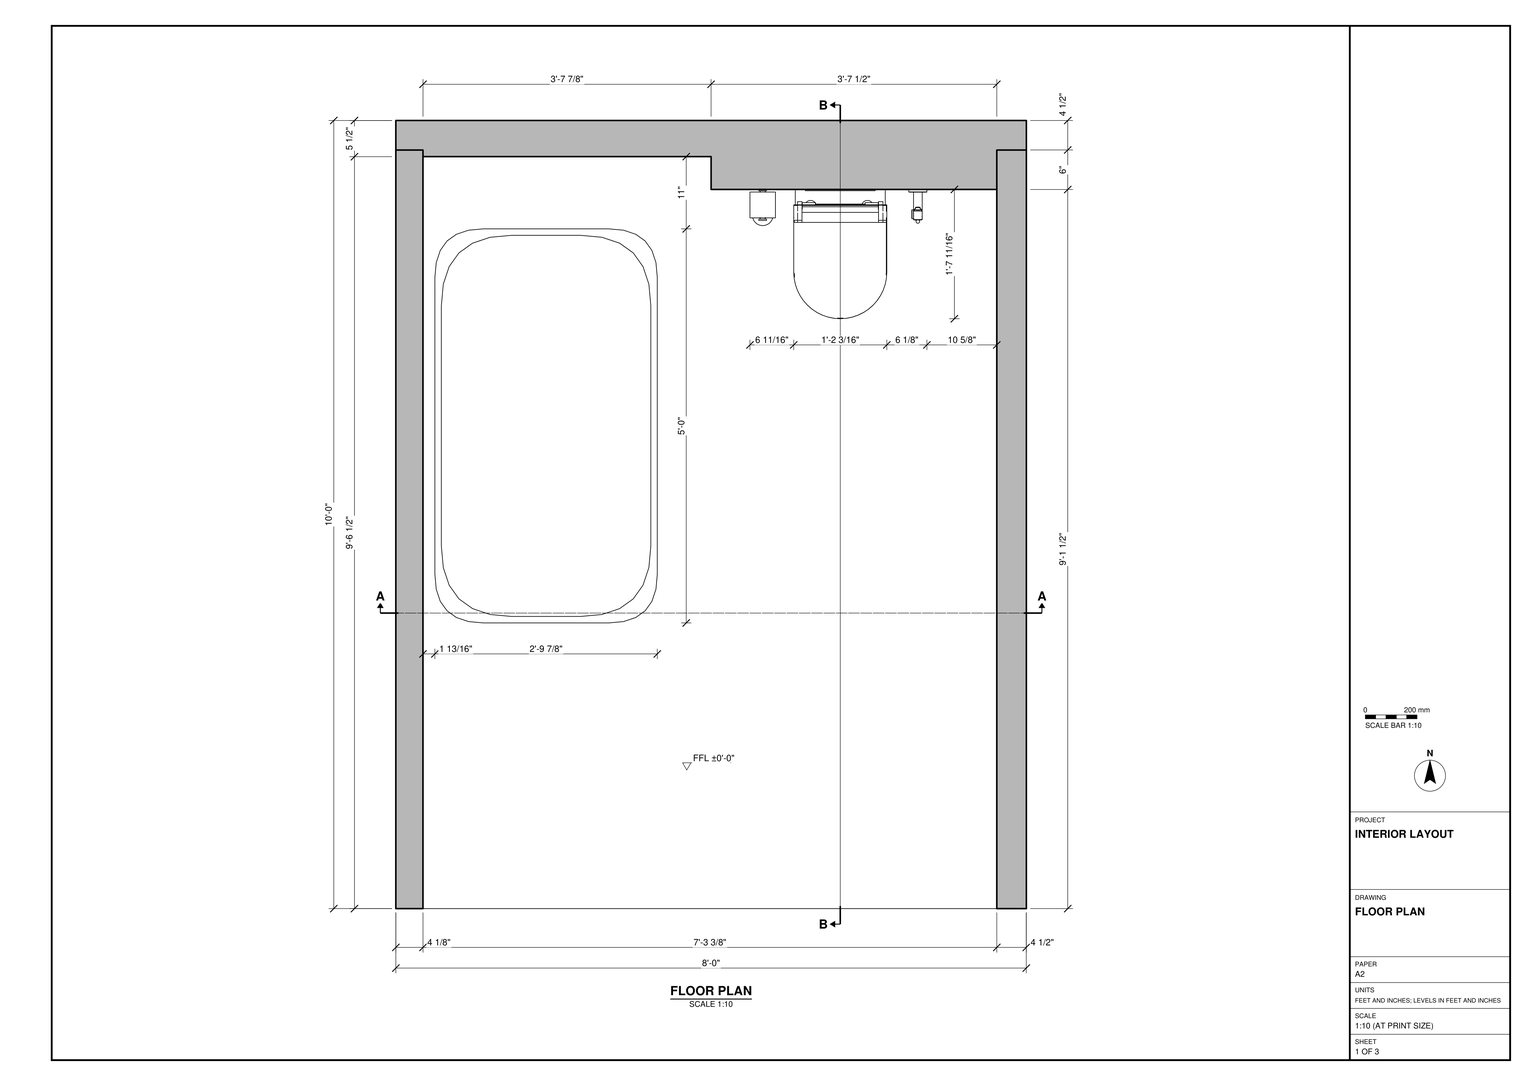
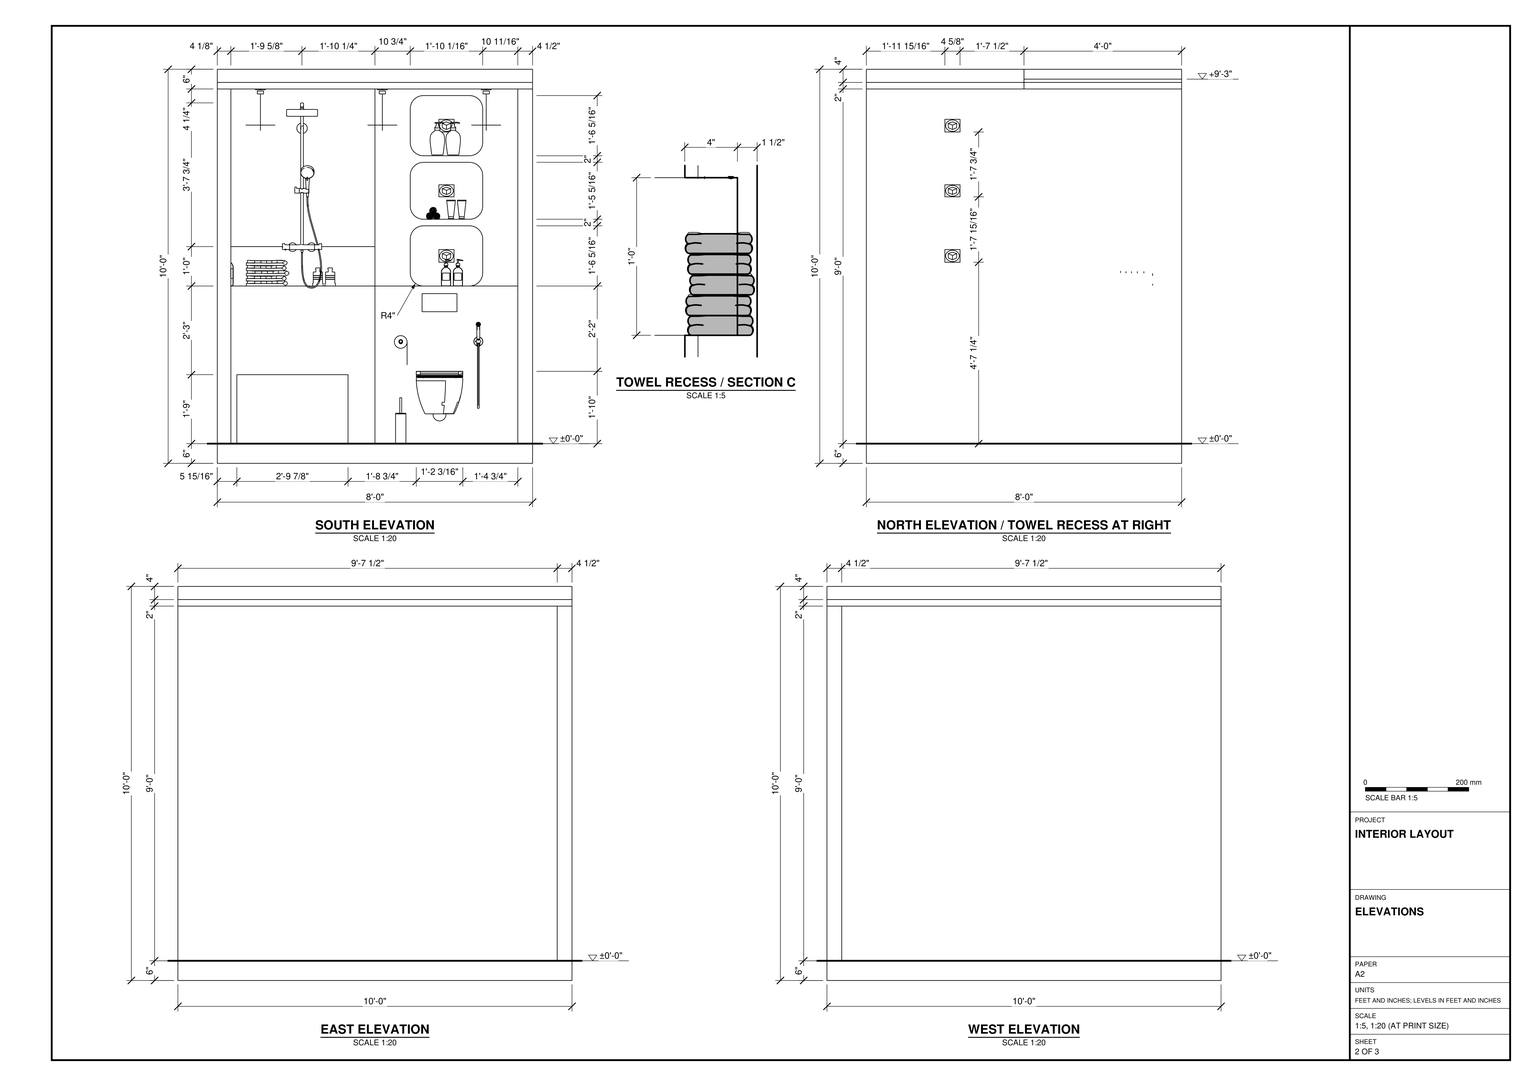
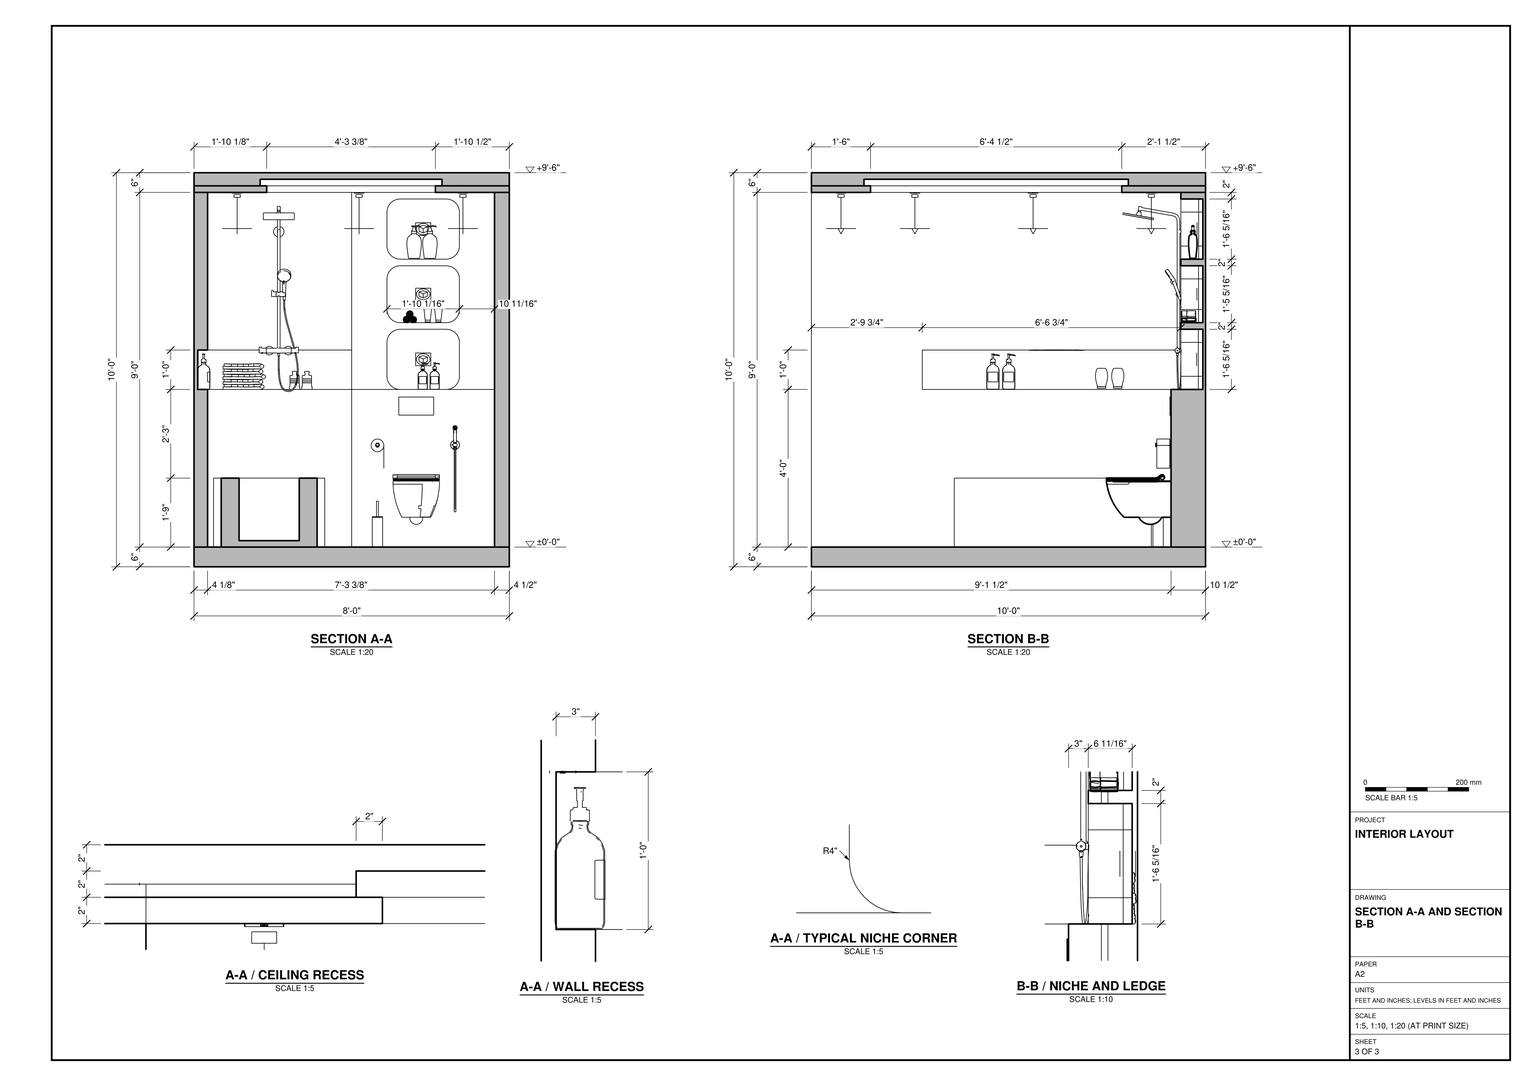
Build the bathroom in SketchUp from task_files/diagram_01.pdf. Work in feet and inches. The room shell is 8'-0" wide, 10'-0" deep and 10'-0" high overall, with the finished floor at ±0'-0". Use the plan for wall thicknesses and fixture positions, and the elevations and sections for heights and recess profiles.

Model the floor slab, the two side walls and the stepped back wall, leaving the front open as drawn. Run the bathtub lengthwise along the left wall, with a rounded rim and a hollow basin. Fit the shower head, hand shower, hose and controls at the back of the tub. Mount the toilet on the projecting part of the back wall to the right, with its flush plate above. Form the three stacked, round-cornered niches above the toilet and the horizontal storage recesses around the bathing area. Place towels and toiletries on the ledges shown. Model the stepped ceiling recess and position the ceiling lights around it as shown in section.

Keep the shell elements, fixtures and individual furniture or joinery pieces in separate groups or components, and use components for repeated parts. Decor and loose items may be any suitable library components. Save one SketchUp model as output_files/bathroom_with_a_bathtub_and_recessed_wall_storage.skp.

# SketchUp Ruby script. Lengths in inches.
U = 1.inch
M = Sketchup.active_model
def pt(a) = Geom::Point3d.new(a.map { |v| v * U })
def face(e, loops, mat)
  f = e.add_face(loops[0].map { |a| pt(a) })
  loops[1..].each { |l| e.add_face(l.map { |a| pt(a) }).erase! }
  f.material = f.back_material = mat if mat
  f
end
# faces: each face lists its corners as indices into pts; further lists are holes
def faces(e, pts, list, mat = nil) = list.each { |f| face(e, (f[0].is_a?(Array) ? f : [f]).map { |l| l.map { |i| pts[i] } }, mat) }
# xy, xz, yz: faces in a plane at the given z, y or x. An outline is a flat list of corners, or four numbers for a rectangle; further outlines are holes
def ring(l) = l.size == 4 ? [[l[0], l[1]], [l[2], l[1]], [l[2], l[3]], [l[0], l[3]]] : l.each_slice(2).to_a
def flat(e, list, mat, &to3) = list.each { |f| face(e, (f[0].is_a?(Array) ? f : [f]).map { |l| ring(l).map { |u, v| to3.(u, v) } }, mat) }
def xy(e, z, list, mat = nil) = flat(e, list, mat) { |x, y| [x, y, z] }
def xz(e, y, list, mat = nil) = flat(e, list, mat) { |x, z| [x, y, z] }
def yz(e, x, list, mat = nil) = flat(e, list, mat) { |y, z| [x, y, z] }
def lines(e, pts, list) = list.each { |a, b| e.add_line(pt(pts[a]), pt(pts[b])) }
# prism: a flat outline (further loops are holes) pulled along v
def prism(e, loops, v, mat = nil)
  f = face(e, loops, mat); d = Geom::Vector3d.new(v.map { |x| x * U })
  f.pushpull(f.normal.samedirection?(d) ? d.length : -d.length)
end
def box(e, o, s, mat = nil) = prism(e, [[o, [o[0] + s[0], o[1], o[2]], [o[0] + s[0], o[1] + s[1], o[2]], [o[0], o[1] + s[1], o[2]]]], [0, 0, s[2]], mat)
def at(x, y, z, deg = 0) = Geom::Transformation.translation(pt([x, y, z])) * Geom::Transformation.rotation(ORIGIN, Z_AXIS, deg.degrees)
def axes(o, x, y, z) = Geom::Transformation.new([*x, 0, *y, 0, *z, 0, *pt(o).to_a, 1])
def part(name) = M.definitions.add(name)
# library, detail: a bought-in or finely detailed component or shape, given as its bounding box
def library(name, o, s) = part(name).tap { |d| box(d.entities, o, s) }
def detail(e, o, s) = box(e.add_group.entities, o, s)
def put(e, d, t, mat = nil) = e.add_instance(d, t).tap { |i| i.material = mat if mat }
def group(e, t, mat = nil) = e.add_group.tap { |g| g.transformation = t; g.material = mat if mat }.entities
root = M.entities
M.materials.add("[Color M00]").color = [255, 255, 255]
c1 = library("Wall-mounted toilet",[0.42,0,-3.5625],[26.94,19.69,45.6875])
c2 = library("Component23",[-347.61,-342.26,23.58],[692.99,696.09,1706.99])
c3 = library("Component7",[-35.53,-35.9,8.59],[73.46,71.43,202.64])
c4 = library("Component24",[-60.51,-34.16,-327.68],[121.07,71.1,439.78])
c5 = library("Component25",[-33.87,-21.9,6.67],[67.74,43.8,171.96])
c6 = library("Component26",[-425.92,-315.64,5.92],[882.4,607.05,1538.44])
c7 = library("Rolled towels",[-0.87,0,-0.63],[7.91,9.92,7.86])
c8 = part("Group237\#1")
p = [[0,0,0],[0,0,-30.17],[-6.71,0,-30.17],[43.68,-54,0],[-43.68,-54,0],[43.68,54,0],
  [43.68,0,0],[-43.68,54,0],[6.71,0,-30.17],[-43.68,0,0],[0,0,-48.84]]
lines(c8.entities,p,[[0,1],[1,2],[3,4],[5,6],[7,5],[1,8],[9,0],[0,6],[8,10],[4,9],[6,3],[2,10],
  [9,7]])
c9 = part("Rectangle Light")
put(c9.entities,c8,at(0,0,0))
c10 = part("Group239\#1")
p = [[0,0,0],[0,0,-8.86],[-4.25,0,-8.86],[27.68,-1,0],[-27.68,-1,0],[27.68,1,0],
  [27.68,0,0],[-27.68,1,0],[4.25,0,-8.86],[-27.68,0,0],[0,0,-14.34]]
lines(c10.entities,p,[[0,1],[1,2],[3,4],[5,6],[7,5],[1,8],[9,0],[0,6],[8,10],[4,9],[6,3],[2,10],
  [9,7]])
c11 = part("Rectangle Light\#1")
put(c11.entities,c10,at(0,0,0))
c12 = part("Group241\#1")
p = [[0,0,0],[0,0,-12.11],[-0.15,0,-12.11],[1,-38.19,0],[-1,-38.19,0],[1,38.19,0],
  [1,0,0],[-1,38.19,0],[0.15,0,-12.11],[-1,0,0],[0,0,-19.6]]
lines(c12.entities,p,[[0,1],[1,2],[3,4],[5,6],[7,5],[1,8],[9,0],[0,6],[8,10],[4,9],[6,3],[2,10],
  [9,7]])
c13 = part("Rectangle Light\#2")
put(c13.entities,c12,at(0,0,0))
c14 = library("Mesh Light",[-0.5,-0.5,-0.1],[1,1,0.2])
c15 = library("Mesh Light\#1",[-0.5,-0.5,-0.1],[1,1,0.2])
c16 = library("Mesh Light\#2",[-0.5,-0.5,-0.1],[1,1,0.2])
c17 = library("Group\#7",[-0.5,-0.5,-0.1],[47.87,2,0.2])
c18 = library("Group\#8",[-0.5,-0.5,-0.1],[2,82.75,0.2])
c19 = library("Group\#10",[-0.5,-0.5,-0.1],[44.87,3.0625,0.2])
c20 = library("Group\#11",[0,0,0],[8.9,8.9,12.63])
c21 = library("组\#90",[0,0,0],[11.96,19.68,56.43])
c22 = library("Group\#190",[0,0,0],[12.05,13.22,9.68])
p = [[4.13,4.17,6],[4.77,4.17,6],[4.77,4.81,6]]
lines(root,p,[[0,1],[1,2],[2,0]])
put(root,c1,axes([53.49,109.5,9.5625],[1,0,0],[0,-1,0],[0,0,1]))
put(root,c2,axes([3.01,88.35,54.26],[0,0.00536,0],[-0.00357,0,0],[0,0,0.00357]))
put(root,c3,axes([73.27,116.69,53.66],[0.04004,0,0],[0,0.04004,0],[0,0,0.04004]))
put(root,c4,axes([71.82,116.09,101.35],[0.03655,0,0],[0,0.03655,0],[0,0,0.02266]))
put(root,c3,axes([69.64,116.69,53.66],[0.04004,0,0],[0,0.04004,0],[0,0,0.04004]))
put(root,c5,axes([71.17,116.24,74.11],[0.03937,0,0],[0,0.03937,0],[0,0,0.03385]))
put(root,c5,axes([74.42,116.24,74.11],[0.03937,0,0],[0,0.03937,0],[0,0,0.03385]))
put(root,c4,axes([67.01,116.09,101.35],[0.03655,0,0],[0,0.03655,0],[0,0,0.02266]))
put(root,c6,axes([30.57,116.08,53.98],[0.0036,0,0],[0,0.0036,0],[0,0,0.0036]))
put(root,c6,axes([34.32,116.08,53.98],[0.0036,0,0],[0,0.0036,0],[0,0,0.0036]))
put(root,c2,axes([3.01,93.28,54.26],[0,0.00536,0],[-0.00357,0,0],[0,0,0.00357]))
put(root,c7,axes([63.66,112.65,74.1],[0.6,0,0],[0,0.444,0],[0,0,0.6]))
put(root,c3,axes([2.94,55.26,53.5625],[0,0.05325,0],[-0.05325,0,0],[0,0,0.05325]))
put(root,c3,axes([2.94,60.08,53.5625],[0,0.05325,0],[-0.05325,0,0],[0,0,0.05325]))
put(root,c9,axes([47.82,0,60],[1,0,0],[0,0,-1],[0,-1,0]))
put(root,c11,axes([47.82,95.5,116.01],[1,0,0],[0,-1,0],[0,0,-1]))
put(root,c11,axes([47.82,17,116.01],[1,0,0],[0,-1,0],[0,0,-1]))
put(root,c13,axes([21.13,56.31,116.01],[1,0,0],[0,-1,0],[0,0,-1]))
put(root,c13,axes([74.5,56.19,116],[1,0,0],[0,-1,0],[0,0,-1]))
g1 = group(root,at(0,0,0))
box(g1,[0,0,0],[96,120,6])
g2 = group(root,at(0,115.5,6))
xy(g2,0,[[48,-6,48,-1,4.13,-1,4.13,0,0,0,0,4.5,96,4.5,96,0,91.5,0,91.5,-6]])
xy(g2,48,[[48,-6,91.5,-6,91.5,-3,76.8125,-3,76.8125,3.6875,62.75,3.6875,62.75,-3,48,-3],[4.13,-1,48,-1,48,3,1.13,3,1.13,0,4.13,0]])
xy(g2,60,[[4.13,-1,4.13,0,1.13,0,1.13,2,48,2,48,-1]])
xy(g2,66.33,[[62.75,-3,76.8125,2.32]])
xy(g2,68.33,[[62.75,-3,76.8125,2.375]])
xy(g2,85.67,[[62.75,-3,76.8125,2.375]])
xy(g2,87.67,[[62.75,-3,76.75,2.41]])
xy(g2,106,[[62.75,-3,76.8125,2.41]])
xy(g2,108,[[48,-3,91.5,-3,91.5,0,96,0,96,4.5,0,4.5,0,0,4.13,0,4.13,-1,48,-1]])
xz(g2,-6,[[48,0,91.5,48]])
xz(g2,-3,[[[48,48,62.75,48,62.23,48.03,61.71,48.14,61.22,48.3,60.75,48.54,60.31,48.83,59.92,49.17,59.58,49.56,59.29,50,59.05,50.47,58.89,50.96,58.78,51.48,58.75,52,58.75,62.33,58.78,62.86,58.89,63.37,59.05,63.86,59.29,64.33,59.58,64.77,59.92,65.16,60.31,65.51,60.75,65.8,61.22,66.03,61.71,66.2,62.23,66.3,62.75,66.33,76.8125,66.33,77.33,66.3,77.85,66.2,78.34,66.03,78.8125,65.8,79.25,65.51,79.64,65.16,79.99,64.77,80.28,64.33,80.51,63.86,80.68,63.37,80.78,62.86,80.8125,62.33,80.8125,52,80.78,51.48,80.68,50.96,80.51,50.47,80.28,50,79.99,49.56,79.64,49.17,79.25,48.83,78.8125,48.54,78.34,48.3,77.85,48.14,77.33,48.03,76.8125,48,91.5,48,91.5,108,48,108],[62.75,87.67,62.23,87.7,61.71,87.8,61.22,87.97,60.75,88.2,60.31,88.49,59.92,88.84,59.58,89.23,59.29,89.67,59.05,90.14,58.89,90.63,58.78,91.14,58.75,91.67,58.75,102,58.78,102.52,58.89,103.04,59.05,103.53,59.29,104,59.58,104.44,59.92,104.83,60.31,105.17,60.75,105.46,61.22,105.7,61.71,105.86,62.23,105.97,62.75,106,76.8125,106,77.33,105.97,77.85,105.86,78.34,105.7,78.8125,105.46,79.25,105.17,79.64,104.83,79.99,104.44,80.28,104,80.51,103.53,80.68,103.04,80.78,102.52,80.8125,102,80.8125,91.73,80.78,91.2,80.67,90.68,80.5,90.17,80.27,89.7,79.97,89.26,79.62,88.86,79.22,88.51,78.78,88.21,78.3,87.98,77.8,87.81,77.28,87.7,76.75,87.67],[62.75,68.33,62.23,68.37,61.71,68.47,61.22,68.64,60.75,68.87,60.31,69.16,59.92,69.5,59.58,69.9,59.29,70.33,59.05,70.8,58.89,71.3,58.78,71.8125,58.75,72.33,58.75,81.67,58.78,82.1875,58.89,82.7,59.05,83.2,59.29,83.67,59.58,84.1,59.92,84.5,60.31,84.84,60.75,85.13,61.22,85.36,61.71,85.53,62.23,85.63,62.75,85.67,76.8125,85.67,77.33,85.63,77.85,85.53,78.34,85.36,78.8125,85.13,79.25,84.84,79.64,84.5,79.99,84.1,80.28,83.67,80.51,83.2,80.68,82.7,80.78,82.1875,80.8125,81.67,80.8125,72.33,80.78,71.8125,80.68,71.3,80.51,70.8,80.28,70.33,79.99,69.9,79.64,69.5,79.25,69.16,78.8125,68.87,78.34,68.64,77.85,68.47,77.33,68.37,76.8125,68.33]]])
xz(g2,-1,[[4.13,0,48,48],[4.13,60,48,108]])
xz(g2,0,[[0,0,4.13,0,4.13,48,1.13,48,1.13,60,4.13,60,4.13,108,0,108],[91.5,0,96,108]])
xz(g2,3,[[1.13,48,48,60]])
xz(g2,3.6875,[[62.75,48,76.8125,48,77.33,48.03,77.85,48.14,78.34,48.3,78.8125,48.54,79.25,48.83,79.64,49.17,79.99,49.56,80.28,50,80.51,50.47,80.68,50.96,80.78,51.48,80.8125,52,80.8125,62.33,80.78,62.86,80.68,63.37,80.51,63.86,80.28,64.33,79.99,64.77,79.64,65.16,79.25,65.51,78.8125,65.8,78.34,66.03,77.85,66.2,77.33,66.3,76.8125,66.33,62.75,66.33,62.23,66.3,61.71,66.2,61.22,66.03,60.75,65.8,60.31,65.51,59.92,65.16,59.58,64.77,59.29,64.33,59.05,63.86,58.89,63.37,58.78,62.86,58.75,62.33,58.75,52,58.78,51.48,58.89,50.96,59.05,50.47,59.29,50,59.58,49.56,59.92,49.17,60.31,48.83,60.75,48.54,61.22,48.3,61.71,48.14,62.23,48.03],[62.75,68.33,76.8125,68.33,77.33,68.37,77.85,68.47,78.34,68.64,78.8125,68.87,79.25,69.16,79.64,69.5,79.99,69.9,80.28,70.33,80.51,70.8,80.68,71.3,80.78,71.8125,80.8125,72.33,80.8125,81.67,80.78,82.1875,80.68,82.7,80.51,83.2,80.28,83.67,79.99,84.1,79.64,84.5,79.25,84.84,78.8125,85.13,78.34,85.36,77.85,85.53,77.33,85.63,76.8125,85.67,62.75,85.67,62.23,85.63,61.71,85.53,61.22,85.36,60.75,85.13,60.31,84.84,59.92,84.5,59.58,84.1,59.29,83.67,59.05,83.2,58.89,82.7,58.78,82.1875,58.75,81.67,58.75,72.33,58.78,71.8125,58.89,71.3,59.05,70.8,59.29,70.33,59.58,69.9,59.92,69.5,60.31,69.16,60.75,68.87,61.22,68.64,61.71,68.47,62.23,68.37],[62.75,87.67,76.75,87.67,77.28,87.7,77.8,87.81,78.3,87.98,78.78,88.21,79.22,88.51,79.62,88.86,79.97,89.26,80.27,89.7,80.5,90.17,80.67,90.68,80.78,91.2,80.8125,91.73,80.8125,102,80.78,102.52,80.68,103.04,80.51,103.53,80.28,104,79.99,104.44,79.64,104.83,79.25,105.17,78.8125,105.46,78.34,105.7,77.85,105.86,77.33,105.97,76.8125,106,62.75,106,62.23,105.97,61.71,105.86,61.22,105.7,60.75,105.46,60.31,105.17,59.92,104.83,59.58,104.44,59.29,104,59.05,103.53,58.89,103.04,58.78,102.52,58.75,102,58.75,91.67,58.78,91.14,58.89,90.63,59.05,90.14,59.29,89.67,59.58,89.23,59.92,88.84,60.31,88.49,60.75,88.2,61.22,87.97,61.71,87.8,62.23,87.7]])
xz(g2,4.5,[[0,0,96,108]])
yz(g2,0,[[0,0,4.5,108]])
yz(g2,1.13,[[0,48,3,60]])
yz(g2,4.13,[[-1,0,0,48],[-1,60,0,108]])
yz(g2,48,[[-6,0,-6,48,-3,48,-3,108,-1,108,-1,60,3,60,3,48,-1,48,-1,0]])
yz(g2,58.75,[[-3,52,2.32,62.33],[-3,72.33,2.375,81.67],[-3,91.67,2.41,102]])
yz(g2,80.8125,[[-3,52,2.32,62.33],[-3,72.33,2.375,81.67],[-3,91.73,2.41,102]])
yz(g2,91.5,[[-6,0,0,0,0,108,-3,108,-3,48,-6,48]])
yz(g2,96,[[0,0,4.5,108]])
p = [[62.23,-3,48.03],[62.23,2.32,48.03],[61.71,2.32,48.14],[61.71,-3,48.14],[62.75,-3,48],[62.75,2.32,48],
  [77.33,-3,48.03],[77.33,2.32,48.03],[76.8125,2.32,48],[76.8125,-3,48],[77.85,-3,48.14],[77.85,2.32,48.14],
  [61.22,2.32,48.3],[61.22,-3,48.3],[78.34,-3,48.3],[78.34,2.32,48.3],[60.75,2.32,48.54],[60.75,-3,48.54],
  [78.8125,-3,48.54],[78.8125,2.32,48.54],[60.31,2.32,48.83],[60.31,-3,48.83],[79.25,-3,48.83],[79.25,2.32,48.83],
  [59.92,2.32,49.17],[59.92,-3,49.17],[79.64,-3,49.17],[79.64,2.32,49.17],[59.58,2.32,49.56],[59.58,-3,49.56],
  [79.99,-3,49.56],[79.99,2.32,49.56],[59.29,2.32,50],[59.29,-3,50],[80.28,-3,50],[80.28,2.32,50],
  [59.05,2.32,50.47],[59.05,-3,50.47],[80.51,-3,50.47],[80.51,2.32,50.47],[58.89,2.32,50.96],[58.89,-3,50.96],
  [80.68,-3,50.96],[80.68,2.32,50.96],[58.78,2.32,51.48],[58.78,-3,51.48],[80.78,-3,51.48],[80.78,2.32,51.48],
  [58.75,2.32,52],[58.75,-3,52],[80.8125,-3,52],[80.8125,2.32,52],[58.75,-3,62.33],[58.75,2.32,62.33],
  [58.78,2.32,62.86],[58.78,-3,62.86],[80.78,-3,62.86],[80.78,2.32,62.86],[80.8125,2.32,62.33],[80.8125,-3,62.33],
  [58.89,2.32,63.37],[58.89,-3,63.37],[80.68,-3,63.37],[80.68,2.32,63.37],[59.05,2.32,63.86],[59.05,-3,63.86],
  [80.51,-3,63.86],[80.51,2.32,63.86],[59.29,2.32,64.33],[59.29,-3,64.33],[80.28,-3,64.33],[80.28,2.32,64.33],
  [59.58,2.32,64.77],[59.58,-3,64.77],[79.99,-3,64.77],[79.99,2.32,64.77],[59.92,2.32,65.16],[59.92,-3,65.16],
  [79.64,-3,65.16],[79.64,2.32,65.16],[60.31,2.32,65.51],[60.31,-3,65.51],[79.25,-3,65.51],[79.25,2.32,65.51],
  [60.75,2.32,65.8],[60.75,-3,65.8],[78.8125,-3,65.8],[78.8125,2.32,65.8],[61.22,2.32,66.03],[61.22,-3,66.03],
  [78.34,-3,66.03],[78.34,2.32,66.03],[61.71,2.32,66.2],[61.71,-3,66.2],[77.85,-3,66.2],[77.85,2.32,66.2],
  [62.23,2.32,66.3],[62.23,-3,66.3],[77.33,-3,66.3],[77.33,2.32,66.3],[62.75,2.32,66.33],[62.75,-3,66.33],
  [76.8125,-3,66.33],[76.8125,2.32,66.33],[62.75,-3,68.33],[62.75,2.375,68.33],[62.23,2.375,68.37],[62.23,-3,68.37],
  [77.33,-3,68.37],[77.33,2.375,68.37],[76.8125,2.375,68.33],[76.8125,-3,68.33],[61.71,2.375,68.47],[61.71,-3,68.47],
  [77.85,-3,68.47],[77.85,2.375,68.47],[61.22,2.375,68.64],[61.22,-3,68.64],[78.34,-3,68.64],[78.34,2.375,68.64],
  [60.75,2.375,68.87],[60.75,-3,68.87],[78.8125,-3,68.87],[78.8125,2.375,68.87],[60.31,2.375,69.16],[60.31,-3,69.16],
  [79.25,-3,69.16],[79.25,2.375,69.16],[59.92,2.375,69.5],[59.92,-3,69.5],[79.64,-3,69.5],[79.64,2.375,69.5],
  [59.58,2.375,69.9],[59.58,-3,69.9],[79.99,-3,69.9],[79.99,2.375,69.9],[59.29,2.375,70.33],[59.29,-3,70.33],
  [80.28,-3,70.33],[80.28,2.375,70.33],[59.05,2.375,70.8],[59.05,-3,70.8],[80.51,-3,70.8],[80.51,2.375,70.8],
  [58.89,2.375,71.3],[58.89,-3,71.3],[80.68,-3,71.3],[80.68,2.375,71.3],[58.78,2.375,71.8125],[58.78,-3,71.8125],
  [80.78,-3,71.8125],[80.78,2.375,71.8125],[58.75,2.375,72.33],[58.75,-3,72.33],[80.8125,-3,72.33],[80.8125,2.375,72.33],
  [58.75,-3,81.67],[58.75,2.375,81.67],[58.78,2.375,82.1875],[58.78,-3,82.1875],[80.78,-3,82.1875],[80.78,2.375,82.1875],
  [80.8125,2.375,81.67],[80.8125,-3,81.67],[58.89,2.375,82.7],[58.89,-3,82.7],[80.68,-3,82.7],[80.68,2.375,82.7],
  [59.05,2.375,83.2],[59.05,-3,83.2],[80.51,-3,83.2],[80.51,2.375,83.2],[59.29,2.375,83.67],[59.29,-3,83.67],
  [80.28,-3,83.67],[80.28,2.375,83.67],[59.58,2.375,84.1],[59.58,-3,84.1],[79.99,-3,84.1],[79.99,2.375,84.1],
  [59.92,2.375,84.5],[59.92,-3,84.5],[79.64,-3,84.5],[79.64,2.375,84.5],[60.31,2.375,84.84],[60.31,-3,84.84],
  [79.25,-3,84.84],[79.25,2.375,84.84],[60.75,2.375,85.13],[60.75,-3,85.13],[78.8125,-3,85.13],[78.8125,2.375,85.13],
  [61.22,2.375,85.36],[61.22,-3,85.36],[78.34,-3,85.36],[78.34,2.375,85.36],[61.71,2.375,85.53],[61.71,-3,85.53],
  [77.85,-3,85.53],[77.85,2.375,85.53],[62.23,2.375,85.63],[62.23,-3,85.63],[77.33,-3,85.63],[77.33,2.375,85.63],
  [62.75,2.375,85.67],[62.75,-3,85.67],[76.8125,-3,85.67],[76.8125,2.375,85.67],[62.23,-3,87.7],[62.23,2.41,87.7],
  [61.71,2.41,87.8],[61.71,-3,87.8],[62.75,-3,87.67],[62.75,2.41,87.67],[77.28,-3,87.7],[77.28,2.41,87.7],
  [76.75,2.41,87.67],[76.75,-3,87.67],[77.8,-3,87.81],[77.8,2.41,87.81],[61.22,2.41,87.97],[61.22,-3,87.97],
  [78.3,-3,87.98],[78.3,2.41,87.98],[60.75,2.41,88.2],[60.75,-3,88.2],[78.78,-3,88.21],[78.78,2.41,88.21],
  [60.31,2.41,88.49],[60.31,-3,88.49],[79.22,-3,88.51],[79.22,2.41,88.51],[59.92,2.41,88.84],[59.92,-3,88.84],
  [79.62,-3,88.86],[79.62,2.41,88.86],[59.58,2.41,89.23],[59.58,-3,89.23],[79.97,-3,89.26],[79.97,2.41,89.26],
  [59.29,2.41,89.67],[59.29,-3,89.67],[80.27,-3,89.7],[80.27,2.41,89.7],[59.05,2.41,90.14],[59.05,-3,90.14],
  [80.5,-3,90.17],[80.5,2.41,90.17],[58.89,2.41,90.63],[58.89,-3,90.63],[80.67,-3,90.68],[80.67,2.41,90.68],
  [58.78,2.41,91.14],[58.78,-3,91.14],[80.78,-3,91.2],[80.78,2.41,91.2],[58.75,2.41,91.67],[58.75,-3,91.67],
  [80.8125,-3,91.73],[80.8125,2.41,91.73],[58.75,-3,102],[58.75,2.41,102],[58.78,2.41,102.52],[58.78,-3,102.52],
  [80.78,-3,102.52],[80.78,2.41,102.52],[80.8125,2.41,102],[80.8125,-3,102],[58.89,2.41,103.04],[58.89,-3,103.04],
  [80.68,-3,103.04],[80.68,2.41,103.04],[59.05,2.41,103.53],[59.05,-3,103.53],[80.51,-3,103.53],[80.51,2.41,103.53],
  [59.29,2.41,104],[59.29,-3,104],[80.28,-3,104],[80.28,2.41,104],[59.58,2.41,104.44],[59.58,-3,104.44],
  [79.99,-3,104.44],[79.99,2.41,104.44],[59.92,2.41,104.83],[59.92,-3,104.83],[79.64,-3,104.83],[79.64,2.41,104.83],
  [60.31,2.41,105.17],[60.31,-3,105.17],[79.25,-3,105.17],[79.25,2.41,105.17],[60.75,2.41,105.46],[60.75,-3,105.46],
  [78.8125,-3,105.46],[78.8125,2.41,105.46],[61.22,2.41,105.7],[61.22,-3,105.7],[78.34,-3,105.7],[78.34,2.41,105.7],
  [61.71,2.41,105.86],[61.71,-3,105.86],[77.85,-3,105.86],[77.85,2.41,105.86],[62.23,2.41,105.97],[62.23,-3,105.97],
  [77.33,-3,105.97],[77.33,2.41,105.97],[62.75,2.41,106],[62.75,-3,106],[76.8125,-3,106],[76.8125,2.41,106]]
faces(g2,p,[[0,1,2,3],[4,5,1,0],[6,7,8,9],[10,11,7,6],[3,2,12,13],[14,15,11,10],[13,12,16,17],[18,19,15,14],
  [17,16,20,21],[22,23,19,18],[21,20,24,25],[26,27,23,22],[25,24,28,29],[30,31,27,26],[29,28,32,33],[34,35,31,30],
  [33,32,36,37],[38,39,35,34],[37,36,40,41],[42,43,39,38],[41,40,44,45],[46,47,43,42],[45,44,48,49],[50,51,47,46],
  [52,53,54,55],[56,57,58,59],[55,54,60,61],[62,63,57,56],[61,60,64,65],[66,67,63,62],[65,64,68,69],[70,71,67,66],
  [69,68,72,73],[74,75,71,70],[73,72,76,77],[78,79,75,74],[77,76,80,81],[82,83,79,78],[81,80,84,85],[86,87,83,82],
  [85,84,88,89],[90,91,87,86],[89,88,92,93],[94,95,91,90],[93,92,96,97],[98,99,95,94],[97,96,100,101],[102,103,99,98],
  [104,105,106,107],[108,109,110,111],[107,106,112,113],[114,115,109,108],[113,112,116,117],[118,119,115,114],[117,116,120,121],[122,123,119,118],
  [121,120,124,125],[126,127,123,122],[125,124,128,129],[130,131,127,126],[129,128,132,133],[134,135,131,130],[133,132,136,137],[138,139,135,134],
  [137,136,140,141],[142,143,139,138],[141,140,144,145],[146,147,143,142],[145,144,148,149],[150,151,147,146],[149,148,152,153],[154,155,151,150],
  [156,157,158,159],[160,161,162,163],[159,158,164,165],[166,167,161,160],[165,164,168,169],[170,171,167,166],[169,168,172,173],[174,175,171,170],
  [173,172,176,177],[178,179,175,174],[177,176,180,181],[182,183,179,178],[181,180,184,185],[186,187,183,182],[185,184,188,189],[190,191,187,186],
  [189,188,192,193],[194,195,191,190],[193,192,196,197],[198,199,195,194],[197,196,200,201],[202,203,199,198],[201,200,204,205],[206,207,203,202],
  [208,209,210,211],[212,213,209,208],[214,215,216,217],[218,219,215,214],[211,210,220,221],[222,223,219,218],[221,220,224,225],[226,227,223,222],
  [225,224,228,229],[230,231,227,226],[229,228,232,233],[234,235,231,230],[233,232,236,237],[238,239,235,234],[237,236,240,241],[242,243,239,238],
  [241,240,244,245],[246,247,243,242],[245,244,248,249],[250,251,247,246],[249,248,252,253],[254,255,251,250],[253,252,256,257],[258,259,255,254],
  [260,261,262,263],[264,265,266,267],[263,262,268,269],[270,271,265,264],[269,268,272,273],[274,275,271,270],[273,272,276,277],[278,279,275,274],
  [277,276,280,281],[282,283,279,278],[281,280,284,285],[286,287,283,282],[285,284,288,289],[290,291,287,286],[289,288,292,293],[294,295,291,290],
  [293,292,296,297],[298,299,295,294],[297,296,300,301],[302,303,299,298],[301,300,304,305],[306,307,303,302],[305,304,308,309],[310,311,307,306]])
g3 = group(g2,at(58.75,2.41,87.67))
xy(g3,0,[[4,0,18,1.28]])
xy(g3,18.33,[[4,0,18.0625,1.28]])
yz(g3,0,[[0,4,1.28,14.33]])
yz(g3,22.0625,[[0,4.0625,1.28,14.33]])
p = [[2.96,1.28,0.14],[2.96,0,0.14],[3.48,0,0.03],[3.48,1.28,0.03],[4,0,0],[4,1.28,0],
  [18,1.28,0],[18,0,0],[18.53,0,0.03],[18.53,1.28,0.03],[19.05,0,0.14],[19.05,1.28,0.14],
  [2.47,1.28,0.3],[2.47,0,0.3],[19.55,0,0.31],[19.55,1.28,0.31],[2,1.28,0.54],[2,0,0.54],
  [20.03,0,0.54],[20.03,1.28,0.54],[1.56,1.28,0.83],[1.56,0,0.83],[20.47,0,0.84],[20.47,1.28,0.84],
  [1.17,1.28,1.17],[1.17,0,1.17],[20.87,0,1.19],[20.87,1.28,1.19],[0.83,1.28,1.56],[0.83,0,1.56],
  [21.22,0,1.59],[21.22,1.28,1.59],[0.54,1.28,2],[0.54,0,2],[21.52,0,2.03],[21.52,1.28,2.03],
  [0.3,1.28,2.47],[0.3,0,2.47],[21.75,0,2.51],[21.75,1.28,2.51],[0.14,1.28,2.96],[0.14,0,2.96],
  [21.92,0,3.01],[21.92,1.28,3.01],[0.03,1.28,3.48],[0.03,0,3.48],[22.03,0,3.53],[22.03,1.28,3.53],
  [0,1.28,4],[0,0,4],[22.0625,0,4.0625],[22.0625,1.28,4.0625],[0.03,1.28,14.86],[0.03,0,14.86],
  [0,0,14.33],[0,1.28,14.33],[22.0625,1.28,14.33],[22.0625,0,14.33],[22.03,0,14.86],[22.03,1.28,14.86],
  [0.14,1.28,15.37],[0.14,0,15.37],[21.93,0,15.37],[21.93,1.28,15.37],[0.3,1.28,15.86],[0.3,0,15.86],
  [21.76,0,15.86],[21.76,1.28,15.86],[0.54,1.28,16.33],[0.54,0,16.33],[21.53,0,16.33],[21.53,1.28,16.33],
  [0.83,1.28,16.77],[0.83,0,16.77],[21.24,0,16.77],[21.24,1.28,16.77],[1.17,1.28,17.16],[1.17,0,17.16],
  [20.89,0,17.16],[20.89,1.28,17.16],[1.56,1.28,17.51],[1.56,0,17.51],[20.5,0,17.51],[20.5,1.28,17.51],
  [2,1.28,17.8],[2,0,17.8],[20.0625,0,17.8],[20.0625,1.28,17.8],[2.47,1.28,18.03],[2.47,0,18.03],
  [19.59,0,18.03],[19.59,1.28,18.03],[2.96,1.28,18.2],[2.96,0,18.2],[19.1,0,18.2],[19.1,1.28,18.2],
  [3.48,1.28,18.3],[3.48,0,18.3],[18.58,0,18.3],[18.58,1.28,18.3],[4,1.28,18.33],[4,0,18.33],
  [18.0625,0,18.33],[18.0625,1.28,18.33]]
faces(g3,p,[[0,1,2,3],[3,2,4,5],[6,7,8,9],[9,8,10,11],[12,13,1,0],[11,10,14,15],[16,17,13,12],[15,14,18,19],
  [20,21,17,16],[19,18,22,23],[24,25,21,20],[23,22,26,27],[28,29,25,24],[27,26,30,31],[32,33,29,28],[31,30,34,35],
  [36,37,33,32],[35,34,38,39],[40,41,37,36],[39,38,42,43],[44,45,41,40],[43,42,46,47],[48,49,45,44],[47,46,50,51],
  [52,53,54,55],[56,57,58,59],[60,61,53,52],[59,58,62,63],[64,65,61,60],[63,62,66,67],[68,69,65,64],[67,66,70,71],
  [72,73,69,68],[71,70,74,75],[76,77,73,72],[75,74,78,79],[80,81,77,76],[79,78,82,83],[84,85,81,80],[83,82,86,87],
  [88,89,85,84],[87,86,90,91],[92,93,89,88],[91,90,94,95],[96,97,93,92],[95,94,98,99],[100,101,97,96],[99,98,102,103]])
put(g3,c14,axes([11.03,0.64,9.17],[23.0625,0,0],[0,2.27665,0],[0,0,19.33333]))
g4 = group(g2,at(58.75,2.375,68.33))
xy(g4,0,[[4,0,18.0625,1.3125]])
xy(g4,17.33,[[4,0,18.0625,1.3125]])
yz(g4,0,[[0,4,1.3125,13.33]])
yz(g4,22.0625,[[0,4,1.3125,13.33]])
p = [[2.96,1.3125,0.14],[2.96,0,0.14],[3.48,0,0.03],[3.48,1.3125,0.03],[4,0,0],[4,1.3125,0],
  [18.0625,1.3125,0],[18.0625,0,0],[18.58,0,0.03],[18.58,1.3125,0.03],[19.1,0,0.14],[19.1,1.3125,0.14],
  [2.47,1.3125,0.3],[2.47,0,0.3],[19.59,0,0.3],[19.59,1.3125,0.3],[2,1.3125,0.54],[2,0,0.54],
  [20.0625,0,0.54],[20.0625,1.3125,0.54],[1.56,1.3125,0.83],[1.56,0,0.83],[20.5,0,0.83],[20.5,1.3125,0.83],
  [1.17,1.3125,1.17],[1.17,0,1.17],[20.89,0,1.17],[20.89,1.3125,1.17],[0.83,1.3125,1.56],[0.83,0,1.56],
  [21.24,0,1.56],[21.24,1.3125,1.56],[0.54,1.3125,2],[0.54,0,2],[21.53,0,2],[21.53,1.3125,2],
  [0.3,1.3125,2.47],[0.3,0,2.47],[21.76,0,2.47],[21.76,1.3125,2.47],[0.14,1.3125,2.96],[0.14,0,2.96],
  [21.93,0,2.96],[21.93,1.3125,2.96],[0.03,1.3125,3.48],[0.03,0,3.48],[22.03,0,3.48],[22.03,1.3125,3.48],
  [0,1.3125,4],[0,0,4],[22.0625,0,4],[22.0625,1.3125,4],[0.03,1.3125,13.86],[0.03,0,13.86],
  [0,0,13.33],[0,1.3125,13.33],[22.0625,1.3125,13.33],[22.0625,0,13.33],[22.03,0,13.86],[22.03,1.3125,13.86],
  [0.14,1.3125,14.37],[0.14,0,14.37],[21.93,0,14.37],[21.93,1.3125,14.37],[0.3,1.3125,14.86],[0.3,0,14.86],
  [21.76,0,14.86],[21.76,1.3125,14.86],[0.54,1.3125,15.33],[0.54,0,15.33],[21.53,0,15.33],[21.53,1.3125,15.33],
  [0.83,1.3125,15.77],[0.83,0,15.77],[21.24,0,15.77],[21.24,1.3125,15.77],[1.17,1.3125,16.16],[1.17,0,16.16],
  [20.89,0,16.16],[20.89,1.3125,16.16],[1.56,1.3125,16.51],[1.56,0,16.51],[20.5,0,16.51],[20.5,1.3125,16.51],
  [2,1.3125,16.8],[2,0,16.8],[20.0625,0,16.8],[20.0625,1.3125,16.8],[2.47,1.3125,17.03],[2.47,0,17.03],
  [19.59,0,17.03],[19.59,1.3125,17.03],[2.96,1.3125,17.2],[2.96,0,17.2],[19.1,0,17.2],[19.1,1.3125,17.2],
  [3.48,1.3125,17.3],[3.48,0,17.3],[18.58,0,17.3],[18.58,1.3125,17.3],[4,1.3125,17.33],[4,0,17.33],
  [18.0625,0,17.33],[18.0625,1.3125,17.33]]
faces(g4,p,[[0,1,2,3],[3,2,4,5],[6,7,8,9],[9,8,10,11],[12,13,1,0],[11,10,14,15],[16,17,13,12],[15,14,18,19],
  [20,21,17,16],[19,18,22,23],[24,25,21,20],[23,22,26,27],[28,29,25,24],[27,26,30,31],[32,33,29,28],[31,30,34,35],
  [36,37,33,32],[35,34,38,39],[40,41,37,36],[39,38,42,43],[44,45,41,40],[43,42,46,47],[48,49,45,44],[47,46,50,51],
  [52,53,54,55],[56,57,58,59],[60,61,53,52],[59,58,62,63],[64,65,61,60],[63,62,66,67],[68,69,65,64],[67,66,70,71],
  [72,73,69,68],[71,70,74,75],[76,77,73,72],[75,74,78,79],[80,81,77,76],[79,78,82,83],[84,85,81,80],[83,82,86,87],
  [88,89,85,84],[87,86,90,91],[92,93,89,88],[91,90,94,95],[96,97,93,92],[95,94,98,99],[100,101,97,96],[99,98,102,103]])
put(g4,c15,axes([11.03,0.66,8.67],[23.0625,0,0],[0,2.3125,0],[0,0,18.33333]))
g5 = group(g2,at(58.75,2.32,48))
xy(g5,18.33,[[4,0,18.0625,1.37]])
yz(g5,0,[[0,4,1.37,14.33]])
yz(g5,22.0625,[[0,4,1.37,14.33]])
p = [[2.96,1.37,0.14],[2.96,0,0.14],[3.48,0,0.03],[3.48,1.37,0.03],[4,0,0],[4,1.37,0],
  [18.0625,1.37,0],[18.0625,0,0],[18.58,0,0.03],[18.58,1.37,0.03],[19.1,0,0.14],[19.1,1.37,0.14],
  [2.47,1.37,0.3],[2.47,0,0.3],[19.59,0,0.3],[19.59,1.37,0.3],[2,1.37,0.54],[2,0,0.54],
  [20.0625,0,0.54],[20.0625,1.37,0.54],[1.56,1.37,0.83],[1.56,0,0.83],[20.5,0,0.83],[20.5,1.37,0.83],
  [1.17,1.37,1.17],[1.17,0,1.17],[20.89,0,1.17],[20.89,1.37,1.17],[0.83,1.37,1.56],[0.83,0,1.56],
  [21.24,0,1.56],[21.24,1.37,1.56],[0.54,1.37,2],[0.54,0,2],[21.53,0,2],[21.53,1.37,2],
  [0.3,1.37,2.47],[0.3,0,2.47],[21.76,0,2.47],[21.76,1.37,2.47],[0.14,1.37,2.96],[0.14,0,2.96],
  [21.93,0,2.96],[21.93,1.37,2.96],[0.03,1.37,3.48],[0.03,0,3.48],[22.03,0,3.48],[22.03,1.37,3.48],
  [0,1.37,4],[0,0,4],[22.0625,0,4],[22.0625,1.37,4],[0.03,1.37,14.86],[0.03,0,14.86],
  [0,0,14.33],[0,1.37,14.33],[22.0625,1.37,14.33],[22.0625,0,14.33],[22.03,0,14.86],[22.03,1.37,14.86],
  [0.14,1.37,15.37],[0.14,0,15.37],[21.93,0,15.37],[21.93,1.37,15.37],[0.3,1.37,15.86],[0.3,0,15.86],
  [21.76,0,15.86],[21.76,1.37,15.86],[0.54,1.37,16.33],[0.54,0,16.33],[21.53,0,16.33],[21.53,1.37,16.33],
  [0.83,1.37,16.77],[0.83,0,16.77],[21.24,0,16.77],[21.24,1.37,16.77],[1.17,1.37,17.16],[1.17,0,17.16],
  [20.89,0,17.16],[20.89,1.37,17.16],[1.56,1.37,17.51],[1.56,0,17.51],[20.5,0,17.51],[20.5,1.37,17.51],
  [2,1.37,17.8],[2,0,17.8],[20.0625,0,17.8],[20.0625,1.37,17.8],[2.47,1.37,18.03],[2.47,0,18.03],
  [19.59,0,18.03],[19.59,1.37,18.03],[2.96,1.37,18.2],[2.96,0,18.2],[19.1,0,18.2],[19.1,1.37,18.2],
  [3.48,1.37,18.3],[3.48,0,18.3],[18.58,0,18.3],[18.58,1.37,18.3],[4,1.37,18.33],[4,0,18.33],
  [18.0625,0,18.33],[18.0625,1.37,18.33]]
faces(g5,p,[[0,1,2,3],[3,2,4,5],[6,7,8,9],[9,8,10,11],[12,13,1,0],[11,10,14,15],[16,17,13,12],[15,14,18,19],
  [20,21,17,16],[19,18,22,23],[24,25,21,20],[23,22,26,27],[28,29,25,24],[27,26,30,31],[32,33,29,28],[31,30,34,35],
  [36,37,33,32],[35,34,38,39],[40,41,37,36],[39,38,42,43],[44,45,41,40],[43,42,46,47],[48,49,45,44],[47,46,50,51],
  [52,53,54,55],[56,57,58,59],[60,61,53,52],[59,58,62,63],[64,65,61,60],[63,62,66,67],[68,69,65,64],[67,66,70,71],
  [72,73,69,68],[71,70,74,75],[76,77,73,72],[75,74,78,79],[80,81,77,76],[79,78,82,83],[84,85,81,80],[83,82,86,87],
  [88,89,85,84],[87,86,90,91],[92,93,89,88],[91,90,94,95],[96,97,93,92],[95,94,98,99],[100,101,97,96],[99,98,102,103]])
put(g5,c16,axes([11.03,0.69,9.17],[23.0625,0,0],[0,2.37057,0],[0,0,19.33333]))
put(g2,c17,at(1.13,2,60))
g6 = group(root,at(91.5,0,6))
box(g6,[0,0,0],[4.5,115.5,108])
g7 = group(root,at(0,0,6))
xy(g7,0,[[0,0,4.13,115.5]])
xy(g7,48,[[1.13,33.75,4.13,115.5]])
xy(g7,60,[[2.13,33.75,4.13,115.5]])
xy(g7,108,[[0,0,4.13,115.5]])
xz(g7,0,[[0,0,4.13,108]])
xz(g7,33.75,[[1.13,48,4.13,60]])
xz(g7,115.5,[[0,0,0,108,4.13,108,4.13,60,1.13,60,1.13,48,4.13,48,4.13,0]])
yz(g7,0,[[0,0,115.5,108]])
yz(g7,1.13,[[33.75,48,115.5,60]])
yz(g7,4.13,[[0,0,115.5,0,115.5,48,33.75,48,33.75,60,115.5,60,115.5,108,0,108]])
put(g7,c18,at(1.13,33.75,60))
g8 = group(root,at(0,0,114))
xy(g8,0,[[[0,0,0,120,48,120,48,114.5,4.13,114.5,4.13,112.5,48,112.5,48,120,96,120,96,0],[22.13,18,73.5,94.5]]])
xy(g8,2,[[[0,0,0,120,48,120,48,114.5,4.13,114.5,4.13,112.5,48,112.5,48,120,96,120,96,0],[20.13,16,75.5,96.5]],[20.13,16,22.13,94.5],[22.13,16,73.5,18],[73.5,16,75.5,94.5],[20.13,94.5,75.5,96.5]])
xy(g8,3,[[4.13,114.5,48,114.5625]])
xy(g8,4,[[20.13,16,75.5,96.5]])
xy(g8,6,[[0,0,96,120]])
xz(g8,0,[[0,0,96,2],[0,2,96,6]])
xz(g8,16,[[20.13,2,75.5,4]])
xz(g8,18,[[22.13,0,73.5,2]])
xz(g8,94.5,[[22.13,0,73.5,2]])
xz(g8,96.5,[[20.13,2,75.5,4]])
xz(g8,112.5,[[4.13,0,48,2],[4.13,2,48,3]])
xz(g8,114.5,[[4.13,0,48,2],[4.13,2,48,3]])
xz(g8,120,[[0,0,48,2],[48,0,96,2],[0,2,48,3],[48,2,96,6],[0,3,48,6]])
yz(g8,0,[[0,0,120,2],[0,2,120,6]])
yz(g8,4.13,[[112.5,0,114.5,2],[112.5,2,114.5,3]])
yz(g8,20.13,[[16,2,96.5,4]])
yz(g8,22.13,[[18,0,94.5,2]])
yz(g8,48,[[112.5,0,114.5,2],[114.5,0,120,2],[112.5,2,114.5,3],[114.5,2,120,3]])
yz(g8,73.5,[[18,0,94.5,2]])
yz(g8,75.5,[[16,2,96.5,4]])
yz(g8,96,[[0,0,120,2],[0,2,120,6]])
put(g8,c19,at(4.13,112.5,3))
put(root,c20,at(8.68,99.05,101.37))
put(root,c20,at(45.81,99.05,101.37))
put(root,c20,at(77.43,99.05,101.37))
put(root,c20,at(77.43,4.55,101.37))
put(root,c20,at(45.81,4.55,101.37))
put(root,c20,at(8.68,4.55,101.37))
put(root,c20,at(8.68,63.05,101.37))
put(root,c20,at(8.68,27.05,101.37))
put(root,c20,at(77.43,63.05,101.37))
put(root,c20,at(77.43,27.05,101.37))
g9 = group(root,at(5.94,43.5,6),"[Color M00]")
xy(g9,0,[[7.39,0,5.13,0.21,3.28,0.82,1.85,1.85,0.82,3.28,0.21,5.13,0,7.39,0,52.61,0.21,54.87,0.82,56.72,1.85,58.15,3.28,59.18,5.13,59.79,7.39,60,26.47,60,28.73,59.79,30.58,59.18,32.01,58.15,33.04,56.72,33.66,54.87,33.86,52.61,33.86,7.39,33.66,5.13,33.04,3.28,32.01,1.85,30.58,0.82,28.73,0.21,26.47,0]])
xy(g9,1.95,[[11.69,0.98,22.17,0.98,25.44,1.28,28.12,2.17,30.2,3.66,31.6875,5.74,32.58,8.42,32.88,11.69,32.88,48.31,32.58,51.58,31.6875,54.26,30.2,56.34,28.12,57.83,25.44,58.72,22.17,59.02,11.69,59.02,8.42,58.72,5.74,57.83,3.66,56.34,2.17,54.26,1.28,51.58,0.98,48.31,0.98,11.69,1.28,8.42,2.17,5.74,3.66,3.66,5.74,2.17,8.42,1.28]])
xy(g9,21,[[[7.39,0,26.47,0,28.73,0.21,30.58,0.82,32.01,1.85,33.04,3.28,33.66,5.13,33.86,7.39,33.86,52.61,33.66,54.87,33.04,56.72,32.01,58.15,30.58,59.18,28.73,59.79,26.47,60,7.39,60,5.13,59.79,3.28,59.18,1.85,58.15,0.82,56.72,0.21,54.87,0,52.61,0,7.39,0.21,5.13,0.82,3.28,1.85,1.85,3.28,0.82,5.13,0.21],[11.69,0.98,8.42,1.28,5.74,2.17,3.66,3.66,2.17,5.74,1.28,8.42,0.98,11.69,0.98,48.31,1.28,51.58,2.17,54.26,3.66,56.34,5.74,57.83,8.42,58.72,11.69,59.02,22.17,59.02,25.44,58.72,28.12,57.83,30.2,56.34,31.6875,54.26,32.58,51.58,32.88,48.31,32.88,11.69,32.58,8.42,31.6875,5.74,30.2,3.66,28.12,2.17,25.44,1.28,22.17,0.98]]])
xz(g9,0,[[7.39,0,26.47,21]])
xz(g9,0.98,[[11.69,1.95,22.17,21]])
xz(g9,59.02,[[11.69,1.95,22.17,21]])
xz(g9,60,[[7.39,0,26.47,21]])
yz(g9,0,[[7.39,0,52.61,21]])
yz(g9,0.98,[[11.69,1.95,48.31,21]])
yz(g9,32.88,[[11.69,1.95,48.31,21]])
yz(g9,33.86,[[7.39,0,52.61,21]])
p = [[7.39,0,0],[7.39,0,21],[5.13,0.21,21],[5.13,0.21,0],[28.73,0.21,0],[28.73,0.21,21],
  [26.47,0,21],[26.47,0,0],[3.28,0.82,21],[3.28,0.82,0],[30.58,0.82,0],[30.58,0.82,21],
  [1.85,1.85,21],[1.85,1.85,0],[32.01,1.85,0],[32.01,1.85,21],[0.82,3.28,21],[0.82,3.28,0],
  [33.04,3.28,0],[33.04,3.28,21],[0.21,5.13,21],[0.21,5.13,0],[33.66,5.13,0],[33.66,5.13,21],
  [0,7.39,21],[0,7.39,0],[33.86,7.39,0],[33.86,7.39,21],[0,52.61,0],[0,52.61,21],
  [0.21,54.87,21],[0.21,54.87,0],[33.86,52.61,21],[33.86,52.61,0],[33.66,54.87,0],[33.66,54.87,21],
  [0.82,56.72,21],[0.82,56.72,0],[33.04,56.72,0],[33.04,56.72,21],[1.85,58.15,21],[1.85,58.15,0],
  [32.01,58.15,0],[32.01,58.15,21],[3.28,59.18,21],[3.28,59.18,0],[30.58,59.18,0],[30.58,59.18,21],
  [5.13,59.79,21],[5.13,59.79,0],[28.73,59.79,0],[28.73,59.79,21],[7.39,60,21],[7.39,60,0],
  [26.47,60,0],[26.47,60,21],[11.69,0.98,21],[11.69,0.98,1.95],[8.42,1.28,1.95],[8.42,1.28,21],
  [25.44,1.28,21],[25.44,1.28,1.95],[22.17,0.98,1.95],[22.17,0.98,21],[5.74,2.17,1.95],[5.74,2.17,21],
  [28.12,2.17,21],[28.12,2.17,1.95],[3.66,3.66,1.95],[3.66,3.66,21],[30.2,3.66,21],[30.2,3.66,1.95],
  [2.17,5.74,1.95],[2.17,5.74,21],[31.6875,5.74,21],[31.6875,5.74,1.95],[1.28,8.42,1.95],[1.28,8.42,21],
  [32.58,8.42,21],[32.58,8.42,1.95],[0.98,11.69,1.95],[0.98,11.69,21],[32.88,11.69,21],[32.88,11.69,1.95],
  [1.28,51.58,1.95],[1.28,51.58,21],[0.98,48.31,21],[0.98,48.31,1.95],[32.58,51.58,21],[32.58,51.58,1.95],
  [32.88,48.31,1.95],[32.88,48.31,21],[2.17,54.26,1.95],[2.17,54.26,21],[31.6875,54.26,21],[31.6875,54.26,1.95],
  [3.66,56.34,1.95],[3.66,56.34,21],[30.2,56.34,21],[30.2,56.34,1.95],[5.74,57.83,1.95],[5.74,57.83,21],
  [28.12,57.83,21],[28.12,57.83,1.95],[8.42,58.72,1.95],[8.42,58.72,21],[25.44,58.72,21],[25.44,58.72,1.95],
  [11.69,59.02,1.95],[11.69,59.02,21],[22.17,59.02,21],[22.17,59.02,1.95]]
faces(g9,p,[[0,1,2,3],[4,5,6,7],[3,2,8,9],[10,11,5,4],[9,8,12,13],[14,15,11,10],[13,12,16,17],[18,19,15,14],
  [17,16,20,21],[22,23,19,18],[21,20,24,25],[26,27,23,22],[28,29,30,31],[32,33,34,35],[31,30,36,37],[35,34,38,39],
  [37,36,40,41],[39,38,42,43],[41,40,44,45],[43,42,46,47],[45,44,48,49],[47,46,50,51],[49,48,52,53],[51,50,54,55],
  [56,57,58,59],[60,61,62,63],[59,58,64,65],[66,67,61,60],[65,64,68,69],[70,71,67,66],[69,68,72,73],[74,75,71,70],
  [73,72,76,77],[78,79,75,74],[77,76,80,81],[82,83,79,78],[84,85,86,87],[88,89,90,91],[92,93,85,84],[94,95,89,88],
  [96,97,93,92],[98,99,95,94],[100,101,97,96],[102,103,99,98],[104,105,101,100],[106,107,103,102],[108,109,105,104],[110,111,107,106]])
put(root,c21,at(19.82,94.82,53.33))
put(root,c22,axes([8.84,119.82,54],[0,-0.44131,0],[0.98171,0,0],[0,0,0.8097]))
